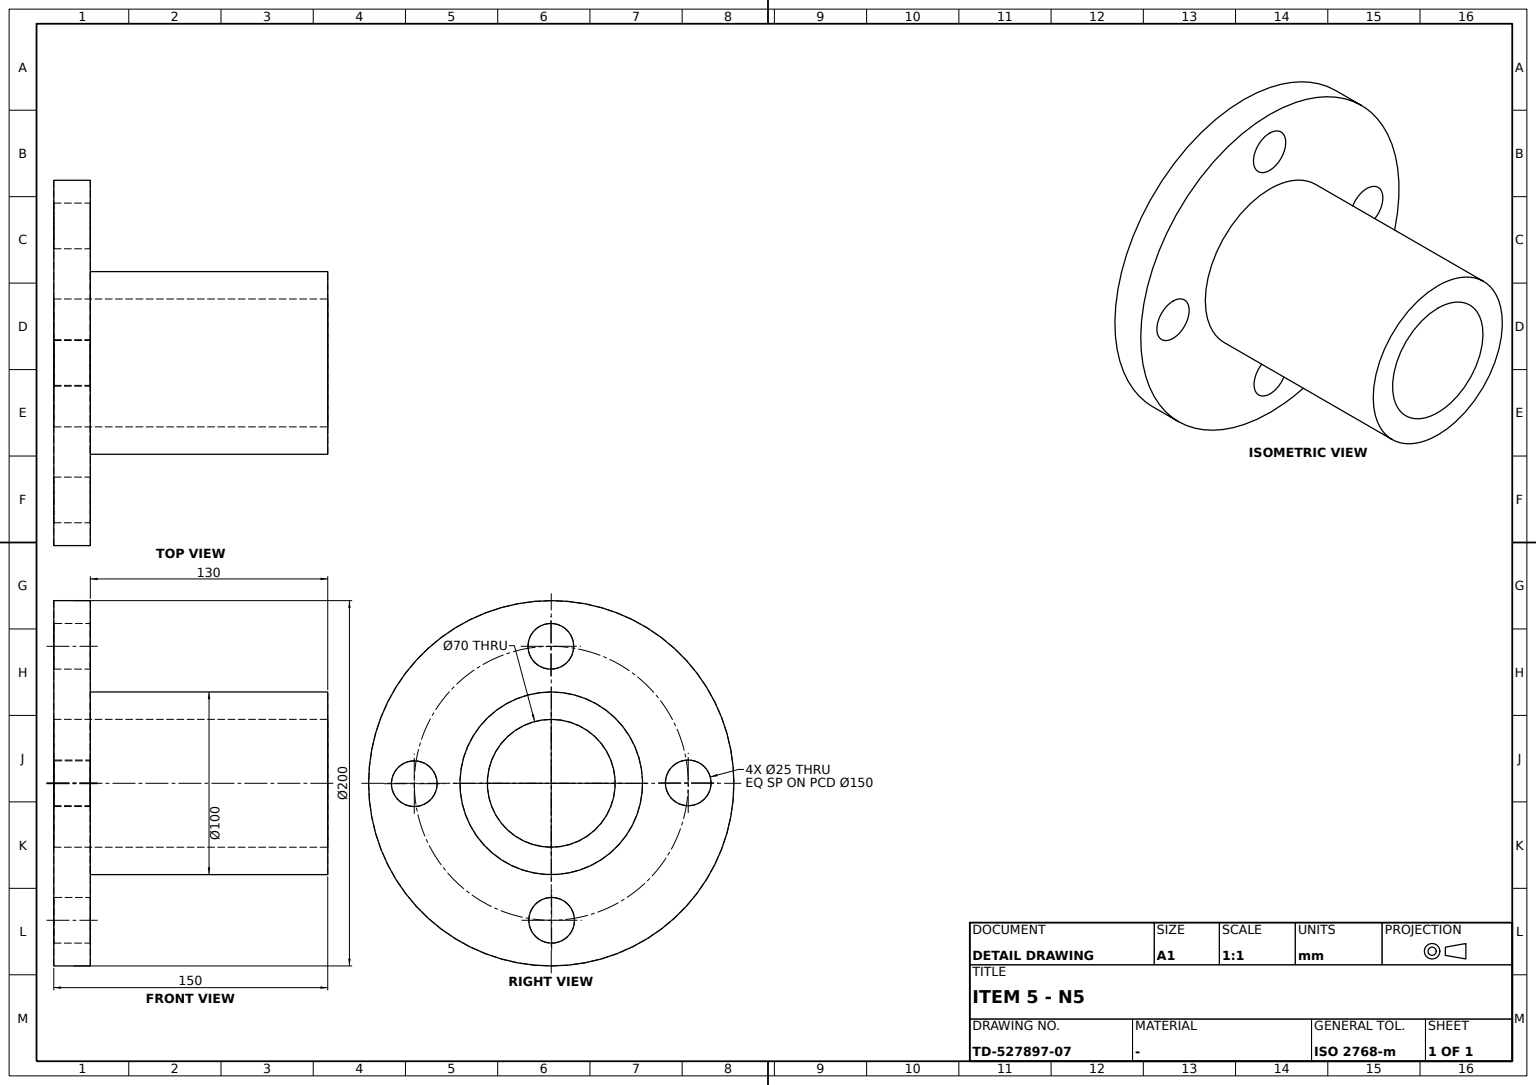
ISO-10303-21;
HEADER;
FILE_DESCRIPTION((''),'2;1');
FILE_NAME('','',(''),(''),'','','');
FILE_SCHEMA(('AUTOMOTIVE_DESIGN'));
ENDSEC;
DATA;
#1=APPLICATION_CONTEXT('');
#2=PRODUCT_CONTEXT('',#1,'mechanical');
#3=PRODUCT('','','',(#2));
#4=PRODUCT_DEFINITION_FORMATION('','',#3);
#5=PRODUCT_DEFINITION_CONTEXT('',#1,'design');
#6=PRODUCT_DEFINITION('','',#4,#5);
#7=PRODUCT_DEFINITION_SHAPE('','',#6);
#8=(LENGTH_UNIT()NAMED_UNIT(*)SI_UNIT(.MILLI.,.METRE.));
#9=(NAMED_UNIT(*)PLANE_ANGLE_UNIT()SI_UNIT($,.RADIAN.));
#10=(NAMED_UNIT(*)SI_UNIT($,.STERADIAN.)SOLID_ANGLE_UNIT());
#11=UNCERTAINTY_MEASURE_WITH_UNIT(LENGTH_MEASURE(0.005),#8,'distance_accuracy_value','');
#12=(GEOMETRIC_REPRESENTATION_CONTEXT(3)GLOBAL_UNCERTAINTY_ASSIGNED_CONTEXT((#11))GLOBAL_UNIT_ASSIGNED_CONTEXT((#8,#9,#10))REPRESENTATION_CONTEXT('',''));
#13=CARTESIAN_POINT('',(-1000.,-1500.,550.));
#14=VERTEX_POINT('',#13);
#15=CARTESIAN_POINT('',(-1000.,-1500.,500.));
#16=DIRECTION('',(0.,1.,0.));
#17=DIRECTION('',(0.,0.,1.));
#18=AXIS2_PLACEMENT_3D('',#15,#16,#17);
#19=CIRCLE('',#18,50.);
#20=EDGE_CURVE('',#14,#14,#19,.T.);
#21=ORIENTED_EDGE('',*,*,#20,.T.);
#22=EDGE_LOOP('',(#21));
#23=FACE_BOUND('',#22,.T.);
#24=CARTESIAN_POINT('',(-1000.,-1500.,535.));
#25=VERTEX_POINT('',#24);
#26=CIRCLE('',#18,35.);
#27=EDGE_CURVE('',#25,#25,#26,.T.);
#28=ORIENTED_EDGE('',*,*,#27,.F.);
#29=EDGE_LOOP('',(#28));
#30=FACE_BOUND('',#29,.T.);
#31=CARTESIAN_POINT('',(0.,-1500.,0.));
#32=DIRECTION('',(-1.,0.,0.));
#33=AXIS2_PLACEMENT_3D('',#31,#16,#32);
#34=PLANE('',#33);
#35=ADVANCED_FACE('',(#23,#30),#34,.T.);
#36=CARTESIAN_POINT('',(-925.00032,-1650.,512.280763));
#37=VERTEX_POINT('',#36);
#38=CARTESIAN_POINT('',(-925.00032,-1650.,499.780763));
#39=AXIS2_PLACEMENT_3D('',#38,#16,#17);
#40=CIRCLE('',#39,12.5);
#41=EDGE_CURVE('',#37,#37,#40,.T.);
#42=ORIENTED_EDGE('',*,*,#41,.T.);
#43=EDGE_LOOP('',(#42));
#44=FACE_BOUND('',#43,.T.);
#45=CARTESIAN_POINT('',(-1074.99968,-1650.,512.719237));
#46=VERTEX_POINT('',#45);
#47=CARTESIAN_POINT('',(-1074.99968,-1650.,500.219237));
#48=AXIS2_PLACEMENT_3D('',#47,#16,#17);
#49=CIRCLE('',#48,12.5);
#50=EDGE_CURVE('',#46,#46,#49,.T.);
#51=ORIENTED_EDGE('',*,*,#50,.T.);
#52=EDGE_LOOP('',(#51));
#53=FACE_BOUND('',#52,.T.);
#54=CARTESIAN_POINT('',(-999.780763,-1650.,587.49968));
#55=VERTEX_POINT('',#54);
#56=CARTESIAN_POINT('',(-999.780763,-1650.,574.99968));
#57=AXIS2_PLACEMENT_3D('',#56,#16,#17);
#58=CIRCLE('',#57,12.5);
#59=EDGE_CURVE('',#55,#55,#58,.T.);
#60=ORIENTED_EDGE('',*,*,#59,.T.);
#61=EDGE_LOOP('',(#60));
#62=FACE_BOUND('',#61,.T.);
#63=CARTESIAN_POINT('',(-1000.,-1650.,535.));
#64=VERTEX_POINT('',#63);
#65=CARTESIAN_POINT('',(-1000.,-1650.,500.));
#66=AXIS2_PLACEMENT_3D('',#65,#16,#17);
#67=CIRCLE('',#66,35.);
#68=EDGE_CURVE('',#64,#64,#67,.T.);
#69=ORIENTED_EDGE('',*,*,#68,.T.);
#70=EDGE_LOOP('',(#69));
#71=FACE_BOUND('',#70,.T.);
#72=CARTESIAN_POINT('',(-1000.,-1650.,600.));
#73=VERTEX_POINT('',#72);
#74=CIRCLE('',#66,100.);
#75=EDGE_CURVE('',#73,#73,#74,.T.);
#76=ORIENTED_EDGE('',*,*,#75,.F.);
#77=EDGE_LOOP('',(#76));
#78=FACE_BOUND('',#77,.T.);
#79=CARTESIAN_POINT('',(-1000.219237,-1650.,437.50032));
#80=VERTEX_POINT('',#79);
#81=CARTESIAN_POINT('',(-1000.219237,-1650.,425.00032));
#82=AXIS2_PLACEMENT_3D('',#81,#16,#17);
#83=CIRCLE('',#82,12.5);
#84=EDGE_CURVE('',#80,#80,#83,.T.);
#85=ORIENTED_EDGE('',*,*,#84,.T.);
#86=EDGE_LOOP('',(#85));
#87=FACE_BOUND('',#86,.T.);
#88=CARTESIAN_POINT('',(0.,-1650.,0.));
#89=AXIS2_PLACEMENT_3D('',#88,#16,#32);
#90=PLANE('',#89);
#91=ADVANCED_FACE('',(#44,#53,#62,#71,#78,#87),#90,.F.);
#92=CARTESIAN_POINT('',(-1000.,-1630.,600.));
#93=VERTEX_POINT('',#92);
#94=CARTESIAN_POINT('',(-1000.,-1630.,500.));
#95=AXIS2_PLACEMENT_3D('',#94,#16,#17);
#96=CIRCLE('',#95,100.);
#97=EDGE_CURVE('',#93,#93,#96,.T.);
#98=ORIENTED_EDGE('',*,*,#97,.F.);
#99=EDGE_LOOP('',(#98));
#100=FACE_BOUND('',#99,.T.);
#101=ORIENTED_EDGE('',*,*,#75,.T.);
#102=EDGE_LOOP('',(#101));
#103=FACE_BOUND('',#102,.T.);
#104=CARTESIAN_POINT('',(-1000.,-1640.,500.));
#105=AXIS2_PLACEMENT_3D('',#104,#16,#32);
#106=CYLINDRICAL_SURFACE('',#105,100.);
#107=ADVANCED_FACE('',(#100,#103),#106,.T.);
#108=CARTESIAN_POINT('',(-999.780763,-1630.,587.49968));
#109=VERTEX_POINT('',#108);
#110=CARTESIAN_POINT('',(-999.780763,-1630.,574.99968));
#111=AXIS2_PLACEMENT_3D('',#110,#16,#17);
#112=CIRCLE('',#111,12.5);
#113=EDGE_CURVE('',#109,#109,#112,.T.);
#114=ORIENTED_EDGE('',*,*,#113,.F.);
#115=EDGE_LOOP('',(#114));
#116=FACE_BOUND('',#115,.T.);
#117=CARTESIAN_POINT('',(-1074.99968,-1630.,512.719237));
#118=VERTEX_POINT('',#117);
#119=CARTESIAN_POINT('',(-1074.99968,-1630.,500.219237));
#120=AXIS2_PLACEMENT_3D('',#119,#16,#17);
#121=CIRCLE('',#120,12.5);
#122=EDGE_CURVE('',#118,#118,#121,.T.);
#123=ORIENTED_EDGE('',*,*,#122,.F.);
#124=EDGE_LOOP('',(#123));
#125=FACE_BOUND('',#124,.T.);
#126=ORIENTED_EDGE('',*,*,#97,.T.);
#127=EDGE_LOOP('',(#126));
#128=FACE_BOUND('',#127,.T.);
#129=CARTESIAN_POINT('',(-1000.219237,-1630.,437.50032));
#130=VERTEX_POINT('',#129);
#131=CARTESIAN_POINT('',(-1000.219237,-1630.,425.00032));
#132=AXIS2_PLACEMENT_3D('',#131,#16,#17);
#133=CIRCLE('',#132,12.5);
#134=EDGE_CURVE('',#130,#130,#133,.T.);
#135=ORIENTED_EDGE('',*,*,#134,.F.);
#136=EDGE_LOOP('',(#135));
#137=FACE_BOUND('',#136,.T.);
#138=CARTESIAN_POINT('',(-925.00032,-1630.,512.280763));
#139=VERTEX_POINT('',#138);
#140=CARTESIAN_POINT('',(-925.00032,-1630.,499.780763));
#141=AXIS2_PLACEMENT_3D('',#140,#16,#17);
#142=CIRCLE('',#141,12.5);
#143=EDGE_CURVE('',#139,#139,#142,.T.);
#144=ORIENTED_EDGE('',*,*,#143,.F.);
#145=EDGE_LOOP('',(#144));
#146=FACE_BOUND('',#145,.T.);
#147=CARTESIAN_POINT('',(-1000.,-1630.,550.));
#148=VERTEX_POINT('',#147);
#149=CIRCLE('',#95,50.);
#150=EDGE_CURVE('',#148,#148,#149,.T.);
#151=ORIENTED_EDGE('',*,*,#150,.F.);
#152=EDGE_LOOP('',(#151));
#153=FACE_BOUND('',#152,.T.);
#154=CARTESIAN_POINT('',(0.,-1630.,0.));
#155=AXIS2_PLACEMENT_3D('',#154,#16,#32);
#156=PLANE('',#155);
#157=ADVANCED_FACE('',(#116,#125,#128,#137,#146,#153),#156,.T.);
#158=ORIENTED_EDGE('',*,*,#113,.T.);
#159=EDGE_LOOP('',(#158));
#160=FACE_BOUND('',#159,.T.);
#161=ORIENTED_EDGE('',*,*,#59,.F.);
#162=EDGE_LOOP('',(#161));
#163=FACE_BOUND('',#162,.T.);
#164=CARTESIAN_POINT('',(-999.780763,-1640.,574.99968));
#165=AXIS2_PLACEMENT_3D('',#164,#16,#32);
#166=CYLINDRICAL_SURFACE('',#165,12.5);
#167=ADVANCED_FACE('',(#160,#163),#166,.F.);
#168=ORIENTED_EDGE('',*,*,#27,.T.);
#169=EDGE_LOOP('',(#168));
#170=FACE_BOUND('',#169,.T.);
#171=ORIENTED_EDGE('',*,*,#68,.F.);
#172=EDGE_LOOP('',(#171));
#173=FACE_BOUND('',#172,.T.);
#174=CARTESIAN_POINT('',(-1000.,-1575.,500.));
#175=AXIS2_PLACEMENT_3D('',#174,#16,#32);
#176=CYLINDRICAL_SURFACE('',#175,35.);
#177=ADVANCED_FACE('',(#170,#173),#176,.F.);
#178=ORIENTED_EDGE('',*,*,#143,.T.);
#179=EDGE_LOOP('',(#178));
#180=FACE_BOUND('',#179,.T.);
#181=ORIENTED_EDGE('',*,*,#41,.F.);
#182=EDGE_LOOP('',(#181));
#183=FACE_BOUND('',#182,.T.);
#184=CARTESIAN_POINT('',(-925.00032,-1640.,499.780763));
#185=AXIS2_PLACEMENT_3D('',#184,#16,#32);
#186=CYLINDRICAL_SURFACE('',#185,12.5);
#187=ADVANCED_FACE('',(#180,#183),#186,.F.);
#188=ORIENTED_EDGE('',*,*,#50,.F.);
#189=EDGE_LOOP('',(#188));
#190=FACE_BOUND('',#189,.T.);
#191=ORIENTED_EDGE('',*,*,#122,.T.);
#192=EDGE_LOOP('',(#191));
#193=FACE_BOUND('',#192,.T.);
#194=CARTESIAN_POINT('',(-1074.99968,-1640.,500.219237));
#195=AXIS2_PLACEMENT_3D('',#194,#16,#32);
#196=CYLINDRICAL_SURFACE('',#195,12.5);
#197=ADVANCED_FACE('',(#190,#193),#196,.F.);
#198=ORIENTED_EDGE('',*,*,#150,.T.);
#199=EDGE_LOOP('',(#198));
#200=FACE_BOUND('',#199,.T.);
#201=ORIENTED_EDGE('',*,*,#20,.F.);
#202=EDGE_LOOP('',(#201));
#203=FACE_BOUND('',#202,.T.);
#204=CYLINDRICAL_SURFACE('',#175,50.);
#205=ADVANCED_FACE('',(#200,#203),#204,.T.);
#206=ORIENTED_EDGE('',*,*,#134,.T.);
#207=EDGE_LOOP('',(#206));
#208=FACE_BOUND('',#207,.T.);
#209=ORIENTED_EDGE('',*,*,#84,.F.);
#210=EDGE_LOOP('',(#209));
#211=FACE_BOUND('',#210,.T.);
#212=CARTESIAN_POINT('',(-1000.219237,-1640.,425.00032));
#213=AXIS2_PLACEMENT_3D('',#212,#16,#32);
#214=CYLINDRICAL_SURFACE('',#213,12.5);
#215=ADVANCED_FACE('',(#208,#211),#214,.F.);
#216=CLOSED_SHELL('',(#35,#91,#107,#157,#167,#177,#187,#197,#205,#215));
#217=MANIFOLD_SOLID_BREP('',#216);
#218=ADVANCED_BREP_SHAPE_REPRESENTATION('',(#217),#12);
#219=SHAPE_DEFINITION_REPRESENTATION(#7,#218);
ENDSEC;
END-ISO-10303-21;
